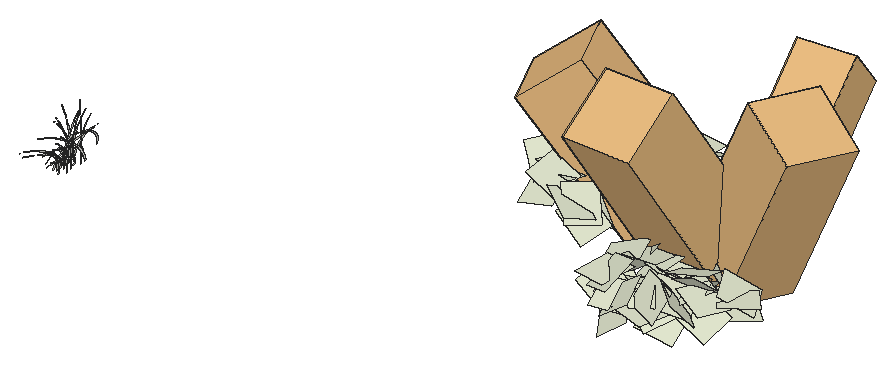
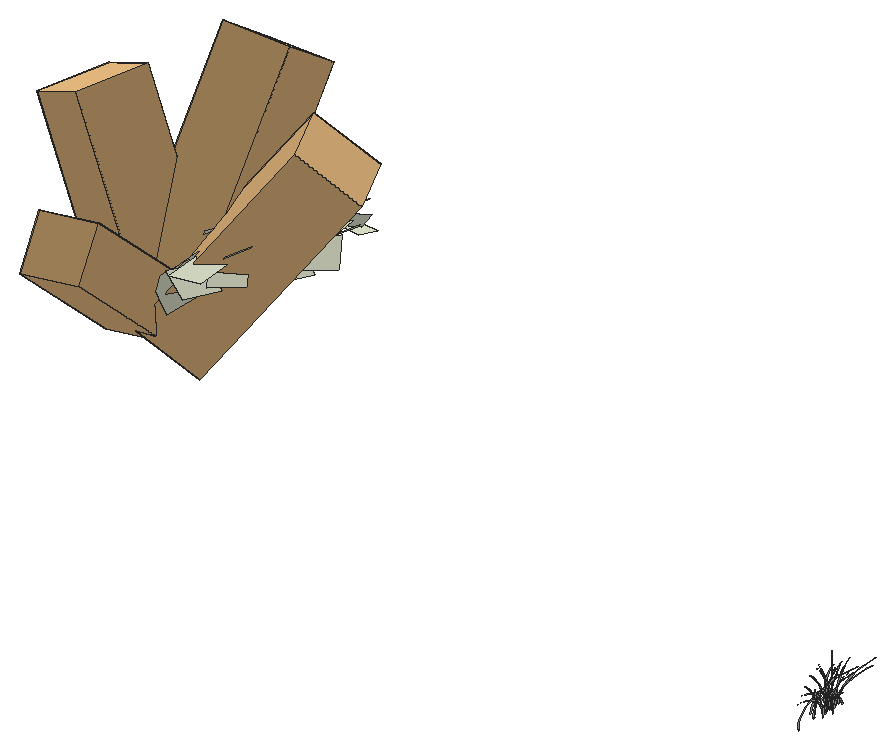
# SketchUp Ruby script. Lengths in inches.
U = 1.inch
M = Sketchup.active_model
def pt(a) = Geom::Point3d.new(a.map { |v| v * U })
def face(e, loops, mat)
  f = e.add_face(loops[0].map { |a| pt(a) })
  loops[1..].each { |l| e.add_face(l.map { |a| pt(a) }).erase! }
  f.material = f.back_material = mat if mat
  f
end
# faces: each face lists its corners as indices into pts; further lists are holes
def faces(e, pts, list, mat = nil) = list.each { |f| face(e, (f[0].is_a?(Array) ? f : [f]).map { |l| l.map { |i| pts[i] } }, mat) }
# xy, xz, yz: faces in a plane at the given z, y or x. An outline is a flat list of corners, or four numbers for a rectangle; further outlines are holes
def ring(l) = l.size == 4 ? [[l[0], l[1]], [l[2], l[1]], [l[2], l[3]], [l[0], l[3]]] : l.each_slice(2).to_a
def flat(e, list, mat, &to3) = list.each { |f| face(e, (f[0].is_a?(Array) ? f : [f]).map { |l| ring(l).map { |u, v| to3.(u, v) } }, mat) }
def xy(e, z, list, mat = nil) = flat(e, list, mat) { |x, y| [x, y, z] }
def xz(e, y, list, mat = nil) = flat(e, list, mat) { |x, z| [x, y, z] }
def yz(e, x, list, mat = nil) = flat(e, list, mat) { |y, z| [x, y, z] }
def lines(e, pts, list) = list.each { |a, b| e.add_line(pt(pts[a]), pt(pts[b])) }
# prism: a flat outline (further loops are holes) pulled along v
def prism(e, loops, v, mat = nil)
  f = face(e, loops, mat); d = Geom::Vector3d.new(v.map { |x| x * U })
  f.pushpull(f.normal.samedirection?(d) ? d.length : -d.length)
end
def box(e, o, s, mat = nil) = prism(e, [[o, [o[0] + s[0], o[1], o[2]], [o[0] + s[0], o[1] + s[1], o[2]], [o[0], o[1] + s[1], o[2]]]], [0, 0, s[2]], mat)
def at(x, y, z, deg = 0) = Geom::Transformation.translation(pt([x, y, z])) * Geom::Transformation.rotation(ORIGIN, Z_AXIS, deg.degrees)
def axes(o, x, y, z) = Geom::Transformation.new([*x, 0, *y, 0, *z, 0, *pt(o).to_a, 1])
def part(name) = M.definitions.add(name)
# library, detail: a bought-in or finely detailed component or shape, given as its bounding box
def library(name, o, s) = part(name).tap { |d| box(d.entities, o, s) }
def detail(e, o, s) = box(e.add_group.entities, o, s)
def put(e, d, t, mat = nil) = e.add_instance(d, t).tap { |i| i.material = mat if mat }
def group(e, t, mat = nil) = e.add_group.tap { |g| g.transformation = t; g.material = mat if mat }.entities
root = M.entities
M.materials.add("Celtis_australis_s cópia1").color = [224, 229, 205]
M.materials.add("bark_cherry").color = [99, 76, 62]
c1 = part("leaf1\#1")
p = [[1.6,6.78,0.04],[-9.34,-4.04,0.02],[2.67,-16.2,2.05],[13.62,-5.38,2.07]]
faces(c1.entities,p,[[0,1,2,3]],"Celtis_australis_s cópia1")
c2 = part("leaf_group1\#1")
put(c2.entities,c1,axes([-0.06,3.68,7.3125],[0.53029,-0.80282,-0.27253],[0.82812,0.42159,0.36943],[-0.18168,-0.42159,0.8884]))
put(c2.entities,c1,axes([6.4375,-3.58,5.23],[1,0,0],[0,0.98927,0.14608],[0,-0.14608,0.98927]))
put(c2.entities,c1,axes([-0.99,3.68,1.22],[0.57591,-0.80282,0.15431],[0.36532,0.42159,0.82994],[-0.73135,-0.42159,0.53609]))
put(c2.entities,c1,axes([18.71,8.59,4.39],[0.33053,0.77491,0.53877],[-0.79988,-0.073,0.5957],[0.50094,-0.62785,0.5957]))
put(c2.entities,c1,axes([13.16,0.76,0.89],[0.89618,0.3501,0.27256],[-0.44248,0.65988,0.60727],[0.03275,-0.66482,0.74628]))
put(c2.entities,c1,axes([4.53,7.98,7.3125],[-0.1927,0.94265,-0.27253],[0.88368,0.28746,0.36943],[-0.42658,0.16964,0.8884]))
put(c2.entities,c1,axes([12.46,21.28,7.16],[0.85019,0.38493,0.35918],[0.30538,-0.91629,0.25914],[-0.42887,0.11063,0.89657]))
put(c2.entities,c1,axes([6.53,15.18,2.59],[0.70711,0.70711,0],[0.5,-0.5,0.70711],[-0.5,0.5,0.70711]))
put(c2.entities,c1,axes([-3.17,8.15,3.46],[-0.03719,0.74973,0.66069],[0.94096,-0.19634,0.27576],[-0.33647,-0.63194,0.69817]))
put(c2.entities,c1,axes([23.03,17.79,4.39],[0.78166,-0.31422,0.53877],[-0.61722,-0.51398,0.5957],[-0.08973,0.79818,0.5957]))
put(c2.entities,c1,axes([14.78,21.52,3.21],[0.67246,-0.04394,0.73882],[-0.28657,-0.93583,0.20517],[-0.6824,0.3497,0.64191]))
put(c2.entities,c1,axes([10.37,-1.8125,9],[0.99279,-0.06448,-0.101],[0.11527,0.74421,0.65792],[0.03275,-0.66482,0.74628]))
put(c2.entities,c1,axes([1.45,16.1875,2.9375],[-0.2106,-0.86579,-0.45394],[0.96054,-0.26957,0.06852],[-0.18168,-0.42159,0.8884]))
c3 = library("branch1\#2",[0,0,0],[33.4,33.29,108.01])
c4 = part("branch2\#1")
p = [[13.74,0.36,0.5],[11.5,11.3125,10.98],[14.125,0.95,0],[14.97,0.95,0.19],[12.12,10.6875,11.67],[15.1,0.36,0.82],
  [11.05,10.4375,11.49],[14.34,0,1.01],[6.08,18.54,23.51],[6.83,18.32,23.89],[6.09,17.93,24.13],[3.27,29.37,34],
  [3.27,29.68,33.56],[3.73,29.59,33.82],[0,43.16,40.74],[0,43.16,40.75],[0.01,43.16,40.75],[5.59,23.2,32.77],
  [4.65,30.48,39.08],[1.92,39.79,43.02],[5.09,28.47,41.41]]
faces(c4.entities,p,[[0,1,2],[2,1,3],[3,4,5],[3,1,4],[6,0,7],[0,6,1],[5,6,7],[6,5,4],
  [6,8,1],[1,9,4],[9,1,8],[8,6,10],[4,10,6],[10,4,9],[10,11,8],[8,12,9],
  [12,8,11],[10,9,11],[13,11,9],[13,9,12],[14,12,11,15],[12,14,16,13],[13,16,15,11]],"bark_cherry")
lines(c4.entities,p,[[17,18],[11,19],[20,17],[17,10]])
g1 = group(root,at(29.53,759.15,-58.625))
p = [[-0.32,0.38,0],[-0.14,0.17,0],[0,0,1.28],[-0.06,0.07,2.5625],[-0.32,0.37,3.82],[-0.77,0.9,5.03],
  [-1.41,1.65,6.15],[-2.21,2.59,7.15],[-3.16,3.7,8.02],[-4.24,4.96,8.72],[-5.41,6.34,9.25],[-6.65,7.79,9.58],
  [-7.93,9.29,9.72],[-9.22,10.79,9.66],[-7.96,9.32,9.67],[-6.71,7.85,9.49],[-5.5,6.44,9.125],[-4.37,5.11,8.58],
  [-3.33,3.89,7.87],[-2.4,2.8125,7.01],[-1.62,1.9,6.02],[-1,1.17,4.92],[-0.55,0.65,3.75],[-0.29,0.33,2.51],
  [-0.21,0.24,1.26]]
faces(g1,p,[[0,1,2,3,4,5,6,7,8,9,10,11,12,13,14,15,16,17,18,19,20,21,22,23,24]])
g2 = group(root,at(25.89,760.17,-58.625))
p = [[-1.7,3.48,4.89],[-1.39,2.85,4.58],[-1.11,2.27,4.24],[-0.86,1.76,3.875],[-0.65,1.33,3.48],[-0.47,0.96,3.08],
  [-0.33,0.68,2.65],[-0.23,0.48,2.22],[-0.18,0.36,1.77],[-0.16,0.33,1.32],[-0.18,0.38,0.875],[-0.25,0.51,0.43],
  [-0.36,0.73,0],[-0.22,0.45,0],[-0.1,0.21,0.44],[-0.03,0.06,0.89],[0,0,1.35],[-0.02,0.04,1.8],
  [-0.08,0.17,2.25],[-0.19,0.4,2.7],[-0.35,0.71,3.125],[-0.54,1.11,3.53],[-0.78,1.6,3.92],[-1.05,2.16,4.27],
  [-1.36,2.79,4.6]]
faces(g2,p,[[0,1,2,3,4,5,6,7,8,9,10,11,12,13,14,15,16,17,18,19,20,21,22,23,24]])
g3 = group(root,at(29.06,755.59,-58.625))
p = [[-0.27,0.46,0],[-0.12,0.21,0],[0,0,1.09],[-0.05,0.08,2.18],[-0.26,0.45,3.25],[-0.64,1.1,4.27],
  [-1.16,2.02,5.22],[-1.82,3.17,6.08],[-2.61,4.53,6.8125],[-3.49,6.07,7.41],[-4.46,7.76,7.86],[-5.48,9.53,8.15],
  [-6.54,11.37,8.26],[-7.59,13.21,8.21],[-6.56,11.4,8.22],[-5.53,9.61,8.07],[-4.53,7.89,7.76],[-3.6,6.26,7.29],
  [-2.74,4.77,6.69],[-1.98,3.44,5.96],[-1.34,2.33,5.12],[-0.82,1.43,4.1875],[-0.45,0.79,3.18],[-0.24,0.41,2.14],
  [-0.17,0.3,1.07]]
faces(g3,p,[[0,1,2,3,4,5,6,7,8,9,10,11,12,13,14,15,16,17,18,19,20,21,22,23,24]])
g4 = group(root,at(27.63,757.12,-58.625))
p = [[-0.51,0.05,0],[-0.23,0.02,0.96],[-0.06,0.01,1.92],[0,0,2.9],[-0.06,0.01,3.87],[-0.22,0.02,4.83],
  [-0.51,0.05,5.79],[-0.9,0.09,6.74],[-1.4,0.14,7.67],[-2,0.2,8.57],[-2.72,0.27,9.46],[-3.53,0.35,10.3125],
  [-4.44,0.44,11.13],[-3.58,0.35,10.3],[-2.82,0.28,9.43],[-2.14,0.21,8.55],[-1.5625,0.15,7.64],[-1.08,0.11,6.71],
  [-0.69,0.07,5.77],[-0.41,0.04,4.82],[-0.23,0.02,3.86],[-0.14,0.01,2.89],[-0.16,0.02,1.92],[-0.29,0.03,0.96]]
faces(g4,p,[[0,1,2,3,4,5,6,7,8,9,10,11,12,13,14,15,16,17,18,19,20,21,22,23]])
g5 = group(root,at(26.74,754.9375,-58.625))
p = [[-2.09,-11.02,8.28],[-2.4,-12.68,8.5],[-2.1,-11.07,8.24],[-1.8,-9.52,7.87],[-1.52,-8.03,7.41],[-1.26,-6.64,6.85],
  [-1.01,-5.35,6.21],[-0.79,-4.18,5.49],[-0.6,-3.14,4.69],[-0.43,-2.25,3.84],[-0.29,-1.51,2.93],[-0.18,-0.93,1.98],
  [-0.1,-0.52,1],[-0.05,-0.29,0],[0,0,0],[-0.04,-0.19,1.03],[-0.11,-0.58,2.03],[-0.22,-1.15,3],
  [-0.36,-1.89,3.93],[-0.53,-2.8,4.8],[-0.73,-3.87,5.61],[-0.96,-5.08,6.33],[-1.22,-6.42,6.97],[-1.49,-7.87,7.51],
  [-1.78,-9.41,7.95]]
faces(g5,p,[[0,1,2,3,4,5,6,7,8,9,10,11,12,13,14,15,16,17,18,19,20,21,22,23,24]])
g6 = group(root,at(26.9375,755.96,-58.625))
p = [[-2.09,-11.02,6.68],[-2.4,-12.68,6.86],[-2.1,-11.07,6.64],[-1.8,-9.52,6.35],[-1.52,-8.03,5.97],[-1.26,-6.64,5.52],
  [-1.01,-5.35,5.01],[-0.79,-4.18,4.42],[-0.6,-3.14,3.79],[-0.43,-2.25,3.1],[-0.29,-1.51,2.36],[-0.18,-0.93,1.6],
  [-0.1,-0.52,0.81],[-0.05,-0.29,0],[0,0,0],[-0.04,-0.19,0.83],[-0.11,-0.58,1.64],[-0.22,-1.15,2.42],
  [-0.36,-1.89,3.17],[-0.53,-2.8,3.875],[-0.73,-3.87,4.52],[-0.96,-5.08,5.11],[-1.22,-6.42,5.62],[-1.49,-7.87,6.06],
  [-1.78,-9.41,6.41]]
faces(g6,p,[[0,1,2,3,4,5,6,7,8,9,10,11,12,13,14,15,16,17,18,19,20,21,22,23,24]])
g7 = group(root,at(26.97,759.05,-58.625))
p = [[-2.3,-4.58,4.26],[-1.86,-3.71,3.98],[-1.47,-2.92,3.6875],[-1.12,-2.22,3.37],[-0.82,-1.625,3.03],[-0.57,-1.13,2.68],
  [-0.375,-0.75,2.31],[-0.24,-0.47,1.93],[-0.15,-0.31,1.54],[-0.13,-0.26,1.15],[-0.17,-0.33,0.76],[-0.26,-0.51,0.38],
  [-0.41,-0.8125,0],[-0.31,-0.61,0],[-0.14,-0.27,0.375],[-0.03,-0.06,0.76],[0.01,0.03,1.15],[0,-0.01,1.54],
  [-0.09,-0.18,1.93],[-0.23,-0.47,2.32],[-0.44,-0.88,2.6875],[-0.71,-1.41,3.05],[-1.03,-2.05,3.39],[-1.41,-2.8,3.7],
  [-1.83,-3.65,3.99]]
faces(g7,p,[[0,1,2,3,4,5,6,7,8,9,10,11,12,13,14,15,16,17,18,19,20,21,22,23,24]])
g8 = group(root,at(28.05,757.3125,-58.625))
p = [[-0.48,0.17,0],[-0.21,0.08,1.22],[-0.05,0.02,2.46],[0,0,3.69],[-0.05,0.02,4.93],[-0.21,0.08,6.17],
  [-0.48,0.17,7.39],[-0.85,0.31,8.6],[-1.32,0.48,9.78],[-1.89,0.6875,10.9375],[-2.57,0.93,12.07],[-3.33,1.21,13.16],
  [-4.19,1.52,14.2],[-3.39,1.23,13.14],[-2.66,0.96,12.04],[-2.02,0.73,10.91],[-1.47,0.53,9.75],[-1.02,0.37,8.5625],
  [-0.66,0.24,7.36],[-0.39,0.14,6.15],[-0.21,0.08,4.92],[-0.14,0.05,3.6875],[-0.15,0.06,2.45],[-0.27,0.1,1.22]]
faces(g8,p,[[0,1,2,3,4,5,6,7,8,9,10,11,12,13,14,15,16,17,18,19,20,21,22,23]])
g9 = group(root,at(27.07,758.11,-58.625))
p = [[-0.22,-0.46,0],[-0.1,-0.21,1.0625],[-0.02,-0.05,2.14],[0,0,3.21],[-0.02,-0.05,4.29],[-0.1,-0.2,5.36],
  [-0.22,-0.46,6.43],[-0.39,-0.8125,7.48],[-0.6,-1.27,8.51],[-0.87,-1.82,9.52],[-1.18,-2.46,10.5],[-1.53,-3.2,11.45],
  [-1.92,-4.03,12.36],[-1.55,-3.25,11.43],[-1.22,-2.55,10.47],[-0.93,-1.94,9.49],[-0.68,-1.42,8.48],[-0.47,-0.98,7.45],
  [-0.3,-0.63,6.4],[-0.18,-0.37,5.35],[-0.1,-0.2,4.28],[-0.0625,-0.13,3.21],[-0.07,-0.15,2.13],[-0.125,-0.26,1.0625]]
faces(g9,p,[[0,1,2,3,4,5,6,7,8,9,10,11,12,13,14,15,16,17,18,19,20,21,22,23]])
g10 = group(root,at(26.16,759.5,-58.625))
p = [[0.03,-0.41,0],[0.01,-0.18,0],[0,0,0.79],[0,-0.07,1.58],[0.03,-0.4,2.36],[0.0625,-0.97,3.11],
  [0.11,-1.77,3.8],[0.18,-2.79,4.42],[0.26,-3.99,4.95],[0.35,-5.34,5.39],[0.44,-6.82,5.71],[0.54,-8.38,5.92],
  [0.65,-9.99,6.01],[0.75,-11.61,5.96],[0.65,-10.02,5.97],[0.55,-8.45,5.86],[0.45,-6.93,5.64],[0.36,-5.5,5.3],
  [0.27,-4.19,4.86],[0.2,-3.03,4.33],[0.13,-2.04,3.72],[0.08,-1.26,3.04],[0.04,-0.69,2.3125],[0.02,-0.36,1.55],
  [0.02,-0.26,0.78]]
faces(g10,p,[[0,1,2,3,4,5,6,7,8,9,10,11,12,13,14,15,16,17,18,19,20,21,22,23,24]])
g11 = group(root,at(26.16,759.5,-58.625))
p = [[0.03,-0.41,0],[0.01,-0.18,0],[0,0,0.79],[0,-0.07,1.58],[0.03,-0.4,2.36],[0.0625,-0.97,3.11],
  [0.11,-1.77,3.8],[0.18,-2.79,4.42],[0.26,-3.99,4.95],[0.35,-5.34,5.39],[0.44,-6.82,5.71],[0.54,-8.38,5.92],
  [0.65,-9.99,6.01],[0.75,-11.61,5.96],[0.65,-10.02,5.97],[0.55,-8.45,5.86],[0.45,-6.93,5.64],[0.36,-5.5,5.3],
  [0.27,-4.19,4.86],[0.2,-3.03,4.33],[0.13,-2.04,3.72],[0.08,-1.26,3.04],[0.04,-0.69,2.3125],[0.02,-0.36,1.55],
  [0.02,-0.26,0.78]]
faces(g11,p,[[0,1,2,3,4,5,6,7,8,9,10,11,12,13,14,15,16,17,18,19,20,21,22,23,24]])
g12 = group(root,at(26.17,769.54,-58.625))
p = [[0.03,-0.46,0],[0.01,-0.21,0],[0,0,0.89],[0.01,-0.08,1.79],[0.03,-0.45,2.67],[0.07,-1.1,3.51],
  [0.13,-2,4.29],[0.2,-3.15,4.99],[0.29,-4.5,5.59],[0.39,-6.04,6.09],[0.5,-7.71,6.45],[0.61,-9.47,6.69],
  [0.73,-11.29,6.79],[0.85,-13.12,6.74],[0.73,-11.33,6.75],[0.62,-9.55,6.625],[0.51,-7.84,6.37],[0.4,-6.22,5.99],
  [0.31,-4.73,5.49],[0.22,-3.42,4.89],[0.15,-2.31,4.2],[0.09,-1.42,3.4375],[0.05,-0.78,2.62],[0.03,-0.41,1.75],
  [0.02,-0.3,0.875]]
faces(g12,p,[[0,1,2,3,4,5,6,7,8,9,10,11,12,13,14,15,16,17,18,19,20,21,22,23,24]])
g13 = group(root,at(28.97,757.5,-58.625))
p = [[-4.78,1.84,4.89],[-3.87,1.49,4.58],[-3.05,1.18,4.24],[-2.32,0.9,3.875],[-1.7,0.66,3.48],[-1.18,0.46,3.08],
  [-0.78,0.3,2.65],[-0.49,0.1875,2.22],[-0.32,0.125,1.77],[-0.27,0.11,1.32],[-0.34,0.13,0.875],[-0.54,0.21,0.43],
  [-0.85,0.33,0],[-0.64,0.25,0],[-0.29,0.11,0.43],[-0.0625,0.02,0.87],[0.03,-0.01,1.32],[-0.01,0,1.77],
  [-0.18,0.07,2.22],[-0.49,0.1875,2.66],[-0.92,0.35,3.09],[-1.47,0.57,3.5],[-2.15,0.83,3.89],[-2.93,1.13,4.26],
  [-3.81,1.47,4.59]]
faces(g13,p,[[0,1,2,3,4,5,6,7,8,9,10,11,12,13,14,15,16,17,18,19,20,21,22,23,24]])
g14 = group(root,at(29.09,761.39,-58.625))
p = [[-4.27,-10.37,9.03],[-4.92,-11.93,9.27],[-4.29,-10.42,8.98],[-3.69,-8.96,8.58],[-3.12,-7.56,8.08],[-2.58,-6.25,7.47],
  [-2.08,-5.04,6.77],[-1.62,-3.94,5.98],[-1.22,-2.96,5.12],[-0.87,-2.12,4.1875],[-0.59,-1.42,3.2],[-0.36,-0.88,2.16],
  [-0.2,-0.49,1.09],[-0.11,-0.27,0],[0,0,0],[-0.08,-0.18,1.12],[-0.22,-0.54,2.22],[-0.44,-1.08,3.28],
  [-0.73,-1.78,4.29],[-1.09,-2.64,5.24],[-1.5,-3.64,6.11],[-1.97,-4.78,6.9],[-2.49,-6.04,7.6],[-3.05,-7.4,8.19],
  [-3.65,-8.85,8.67]]
faces(g14,p,[[0,1,2,3,4,5,6,7,8,9,10,11,12,13,14,15,16,17,18,19,20,21,22,23,24]])
g15 = group(root,at(27.12,759.32,-58.625))
yz(g15,0,[[0.08,0,0,0.81,0.11,1.62,0.4,2.41,0.87,3.16,1.5,3.85,2.29,4.48,3.22,5.03,4.26,5.47,5.39,5.82,6.58,6.04,7.82,6.15,9.07,6.14,7.85,6.1,6.65,5.95,5.49,5.7,4.4,5.34,3.4,4.89,2.5,4.36,1.72,3.74,1.08,3.07,0.58,2.34,0.25,1.58,0.08,0.79]])
g16 = group(root,at(27.12,756.66,-58.625))
yz(g16,0,[[0.51,0,0.23,1.1,0.06,2.21,0,3.33,0.06,4.44,0.23,5.56,0.51,6.66,0.9,7.74,1.4,8.8125,2.01,9.85,2.73,10.87,3.55,11.85,4.46,12.8,3.6,11.84,2.83,10.84,2.15,9.82,1.57,8.78,1.08,7.71,0.7,6.63,0.41,5.54,0.23,4.43,0.14,3.32,0.16,2.21,0.29,1.1]])
g17 = group(root,at(27.12,758.1,-58.625))
yz(g17,0,[[0.07,0,0,1.08,0.03,2.17,0.16,3.25,0.39,4.32,0.72,5.38,1.16,6.43,1.6875,7.46,2.31,8.46,3.04,9.4375,3.85,10.38,4.75,11.29,5.73,12.17,4.82,11.27,3.98,10.34,3.22,9.39,2.53,8.4,1.93,7.4,1.41,6.38,0.97,5.34,0.62,4.29,0.35,3.22,0.17,2.15,0.08,1.08]])
g18 = group(root,at(27.12,761.76,-58.625))
yz(g18,0,[[0.5,0,0.23,0.89,0.0625,1.81,0,2.74,0.04,3.66,0.19,4.58,0.44,5.48,0.79,6.35,1.24,7.18,1.78,7.96,2.4,8.69,3.1,9.35,3.875,9.94,3.17,9.3125,2.53,8.62,1.96,7.875,1.48,7.08,1.07,6.25,0.76,5.39,0.53,4.5,0.4,3.6,0.36,2.69,0.42,1.78,0.57,0.88,0.8125,0]])
g19 = group(root,at(26.76,753.74,-58.625))
p = [[0.78,-3.8,3.62],[0.64,-3.1,3.39],[0.51,-2.47,3.14],[0.4,-1.92,2.86],[0.3,-1.44,2.58],[0.22,-1.05,2.27],
  [0.15,-0.74,1.96],[0.11,-0.52,1.64],[0.08,-0.39,1.31],[0.07,-0.36,0.98],[0.08,-0.41,0.65],[0.12,-0.56,0.32],
  [0.16,-0.79,0],[0.1,-0.49,0],[0.05,-0.22,0.33],[0.01,-0.0625,0.66],[0,0,1],[0.01,-0.04,1.33],
  [0.04,-0.1875,1.67],[0.09,-0.43,1.99],[0.16,-0.77,2.31],[0.25,-1.21,2.61],[0.36,-1.74,2.9],[0.49,-2.35,3.16],
  [0.63,-3.04,3.4]]
faces(g19,p,[[0,1,2,3,4,5,6,7,8,9,10,11,12,13,14,15,16,17,18,19,20,21,22,23,24]])
g20 = group(root,at(26.04,752.64,-58.625))
p = [[2.09,11.02,6.68],[2.4,12.68,6.86],[2.1,11.07,6.64],[1.8,9.52,6.35],[1.52,8.03,5.97],[1.26,6.64,5.52],
  [1.01,5.35,5.01],[0.79,4.18,4.42],[0.6,3.14,3.79],[0.43,2.25,3.1],[0.29,1.51,2.36],[0.18,0.93,1.6],
  [0.1,0.52,0.81],[0.05,0.29,0],[0,0,0],[0.04,0.19,0.83],[0.11,0.58,1.64],[0.22,1.15,2.42],
  [0.36,1.89,3.17],[0.53,2.8,3.875],[0.73,3.87,4.52],[0.96,5.08,5.11],[1.22,6.42,5.62],[1.49,7.87,6.06],
  [1.78,9.41,6.41]]
faces(g20,p,[[0,1,2,3,4,5,6,7,8,9,10,11,12,13,14,15,16,17,18,19,20,21,22,23,24]])
g21 = group(root,at(26.86,763.03,-58.625))
p = [[0.89,-4.29,4.09],[0.72,-3.5,3.83],[0.58,-2.8,3.54],[0.45,-2.17,3.24],[0.34,-1.63,2.91],[0.25,-1.1875,2.57],
  [0.17,-0.84,2.22],[0.12,-0.59,1.85],[0.09,-0.44,1.48],[0.08,-0.4,1.11],[0.1,-0.46,0.73],[0.13,-0.63,0.36],
  [0.19,-0.9,0],[0.11,-0.55,0],[0.05,-0.25,0.37],[0.01,-0.07,0.74],[0,0,1.125],[0.01,-0.05,1.51],
  [0.04,-0.21,1.88],[0.1,-0.49,2.25],[0.18,-0.875,2.61],[0.28,-1.37,2.95],[0.41,-1.96,3.27],[0.55,-2.65,3.57],
  [0.71,-3.43,3.84]]
faces(g21,p,[[0,1,2,3,4,5,6,7,8,9,10,11,12,13,14,15,16,17,18,19,20,21,22,23,24]])
g22 = group(root,at(27.02,757.67,-58.625))
p = [[0.1,-0.5,0],[0.05,-0.22,0.8125],[0.01,-0.06,1.64],[0,0,2.46],[0.01,-0.05,3.29],[0.05,-0.22,4.11],
  [0.1,-0.5,4.92],[0.18,-0.88,5.73],[0.28,-1.375,6.52],[0.41,-1.97,7.29],[0.55,-2.67,8.04],[0.72,-3.47,8.76],
  [0.9,-4.37,9.46],[0.73,-3.53,8.75],[0.57,-2.77,8.02],[0.44,-2.11,7.27],[0.32,-1.54,6.49],[0.22,-1.0625,5.7],
  [0.14,-0.68,4.9],[0.08,-0.4,4.09],[0.05,-0.22,3.28],[0.03,-0.14,2.46],[0.03,-0.16,1.63],[0.06,-0.28,0.81]]
faces(g22,p,[[0,1,2,3,4,5,6,7,8,9,10,11,12,13,14,15,16,17,18,19,20,21,22,23]])
g23 = group(root,at(24.88,758.11,-58.625))
p = [[0.21,-0.49,0],[0.09,-0.22,0],[0,0,0.95],[0.04,-0.09,1.9],[0.21,-0.48,2.83],[0.5,-1.17,3.72],
  [0.91,-2.14,4.55],[1.43,-3.36,5.29],[2.05,-4.81,5.93],[2.75,-6.45,6.45],[3.51,-8.23,6.84],[4.31,-10.12,7.09],
  [5.14,-12.06,7.1875],[5.98,-14.01,7.14],[5.16,-12.1,7.15],[4.35,-10.2,7.02],[3.57,-8.37,6.75],[2.83,-6.64,6.35],
  [2.16,-5.06,5.82],[1.56,-3.65,5.18],[1.05,-2.47,4.45],[0.65,-1.52,3.64],[0.36,-0.84,2.77],[0.19,-0.43,1.86],
  [0.14,-0.32,0.93]]
faces(g23,p,[[0,1,2,3,4,5,6,7,8,9,10,11,12,13,14,15,16,17,18,19,20,21,22,23,24]])
g24 = group(root,at(25.37,756.47,-58.625))
p = [[5.05,-0.84,3.62],[4.09,-0.68,3.39],[3.22,-0.54,3.14],[2.46,-0.41,2.86],[1.8,-0.3,2.58],[1.25,-0.21,2.27],
  [0.82,-0.14,1.96],[0.52,-0.09,1.64],[0.34,-0.06,1.31],[0.29,-0.05,0.98],[0.36,-0.06,0.65],[0.57,-0.09,0.32],
  [0.9,-0.15,0],[0.68,-0.11,0],[0.3,-0.05,0.32],[0.07,-0.01,0.64],[-0.03,0.01,0.98],[0.01,0,1.31],
  [0.19,-0.03,1.64],[0.52,-0.09,1.97],[0.97,-0.16,2.28],[1.56,-0.26,2.59],[2.27,-0.375,2.88],[3.09,-0.51,3.15],
  [4.03,-0.67,3.39]]
faces(g24,p,[[0,1,2,3,4,5,6,7,8,9,10,11,12,13,14,15,16,17,18,19,20,21,22,23,24]])
g25 = group(root,at(27.31,756.27,-58.625))
p = [[1.16,-5.61,9],[0.98,-4.72,8.33],[0.81,-3.9,7.65],[0.65,-3.15,6.94],[0.51,-2.48,6.22],[0.39,-1.89,5.47],
  [0.28,-1.375,4.72],[0.2,-0.95,3.95],[0.125,-0.6,3.17],[0.07,-0.34,2.38],[0.03,-0.17,1.59],[0.02,-0.08,0.8],
  [0.02,-0.07,0],[0,0,0.8],[0.01,-0.03,1.6],[0.03,-0.15,2.4],[0.08,-0.38,3.19],[0.15,-0.71,3.98],
  [0.23,-1.13,4.75],[0.34,-1.65,5.51],[0.47,-2.27,6.26],[0.61,-2.97,6.98],[0.78,-3.77,7.68],[0.96,-4.65,8.35]]
faces(g25,p,[[0,1,2,3,4,5,6,7,8,9,10,11,12,13,14,15,16,17,18,19,20,21,22,23]])
g26 = group(root,at(28.05,752.68,-58.625))
p = [[0.78,-3.8,7.35],[0.64,-3.1,6.89],[0.51,-2.47,6.375],[0.4,-1.92,5.82],[0.3,-1.44,5.24],[0.22,-1.05,4.625],
  [0.15,-0.74,3.99],[0.11,-0.52,3.33],[0.08,-0.39,2.66],[0.07,-0.36,1.99],[0.08,-0.41,1.32],[0.12,-0.56,0.65],
  [0.16,-0.79,0],[0.1,-0.49,0],[0.05,-0.22,0.66],[0.01,-0.0625,1.34],[0,0,2.02],[0.01,-0.04,2.71],
  [0.04,-0.1875,3.39],[0.09,-0.43,4.05],[0.16,-0.77,4.7],[0.25,-1.21,5.31],[0.36,-1.74,5.89],[0.49,-2.35,6.43],
  [0.63,-3.04,6.92]]
faces(g26,p,[[0,1,2,3,4,5,6,7,8,9,10,11,12,13,14,15,16,17,18,19,20,21,22,23,24]])
g27 = group(root,at(26.24,756.84,-58.625))
p = [[0.51,-0.07,0],[0.23,-0.03,0.9],[0.06,-0.01,1.82],[0,0,2.73],[0.06,-0.01,3.65],[0.22,-0.03,4.56],
  [0.5,-0.07,5.46],[0.89,-0.13,6.36],[1.39,-0.2,7.23],[1.99,-0.29,8.09],[2.7,-0.39,8.92],[3.51,-0.51,9.73],
  [4.42,-0.64,10.5],[3.5625,-0.51,9.72],[2.8,-0.4,8.9],[2.13,-0.31,8.0625],[1.55,-0.22,7.21],[1.07,-0.15,6.33],
  [0.69,-0.1,5.44],[0.41,-0.06,4.54],[0.22,-0.03,3.64],[0.14,-0.02,2.73],[0.16,-0.02,1.8125],[0.28,-0.04,0.9]]
faces(g27,p,[[0,1,2,3,4,5,6,7,8,9,10,11,12,13,14,15,16,17,18,19,20,21,22,23]])
g28 = group(root,at(27.55,755.0625,-58.625))
p = [[1.84,-8.88,4.54],[1.59,-7.6875,4.51],[1.35,-6.51,4.4],[1.11,-5.38,4.21],[0.89,-4.31,3.95],[0.6875,-3.33,3.62],
  [0.51,-2.44,3.22],[0.35,-1.68,2.77],[0.22,-1.05,2.27],[0.12,-0.57,1.73],[0.05,-0.24,1.17],[0.02,-0.08,0.59],
  [0.02,-0.08,0],[0,0,0.6],[0.02,-0.1,1.2],[0.08,-0.39,1.78],[0.18,-0.85,2.33],[0.3,-1.47,2.85],
  [0.46,-2.24,3.3125],[0.65,-3.15,3.72],[0.86,-4.17,4.05],[1.09,-5.28,4.3],[1.33,-6.45,4.47],[1.58,-7.66,4.55]]
faces(g28,p,[[0,1,2,3,4,5,6,7,8,9,10,11,12,13,14,15,16,17,18,19,20,21,22,23]])
g29 = group(root,at(28.93,754.48,-58.625))
p = [[2.37,-3.07,3.62],[1.9375,-2.51,3.39],[1.54,-2,3.14],[1.2,-1.55,2.86],[0.9,-1.17,2.58],[0.66,-0.85,2.27],
  [0.46,-0.6,1.96],[0.33,-0.42,1.64],[0.25,-0.32,1.31],[0.22,-0.29,0.98],[0.26,-0.33,0.65],[0.35,-0.45,0.32],
  [0.5,-0.64,0],[0.3,-0.39,0],[0.14,-0.18,0.33],[0.04,-0.05,0.66],[0,0,1],[0.03,-0.03,1.33],
  [0.12,-0.15,1.67],[0.27,-0.35,1.99],[0.48,-0.625,2.31],[0.76,-0.98,2.61],[1.09,-1.41,2.9],[1.47,-1.9,3.16],
  [1.9,-2.45,3.4]]
faces(g29,p,[[0,1,2,3,4,5,6,7,8,9,10,11,12,13,14,15,16,17,18,19,20,21,22,23,24]])
g30 = group(root,at(25.99,756.8125,-58.625))
p = [[0.3125,-0.39,0],[0.14,-0.17,0],[0,0,1.11],[0.06,-0.07,2.23],[0.31,-0.38,3.33],[0.74,-0.93,4.375],
  [1.36,-1.69,5.35],[2.13,-2.66,6.22],[3.05,-3.8,6.97],[4.08,-5.09,7.59],[5.21,-6.5,8.05],[6.41,-8,8.34],
  [7.64,-9.53,8.46],[8.87,-11.07,8.4],[7.66,-9.5625,8.41],[6.46,-8.0625,8.26],[5.3,-6.61,7.9375],[4.2,-5.25,7.47],
  [3.2,-4,6.85],[2.3125,-2.89,6.1],[1.5625,-1.95,5.24],[0.96,-1.2,4.28],[0.53,-0.66,3.26],[0.27,-0.34,2.1875],
  [0.2,-0.25,1.09]]
faces(g30,p,[[0,1,2,3,4,5,6,7,8,9,10,11,12,13,14,15,16,17,18,19,20,21,22,23,24]])
g31 = group(root,at(25.99,756.8125,-58.625))
p = [[0.3125,-0.39,0],[0.14,-0.17,0],[0,0,1.11],[0.06,-0.07,2.23],[0.31,-0.38,3.33],[0.74,-0.93,4.375],
  [1.36,-1.69,5.35],[2.13,-2.66,6.22],[3.05,-3.8,6.97],[4.08,-5.09,7.59],[5.21,-6.5,8.05],[6.41,-8,8.34],
  [7.64,-9.53,8.46],[8.87,-11.07,8.4],[7.66,-9.5625,8.41],[6.46,-8.0625,8.26],[5.3,-6.61,7.9375],[4.2,-5.25,7.47],
  [3.2,-4,6.85],[2.3125,-2.89,6.1],[1.5625,-1.95,5.24],[0.96,-1.2,4.28],[0.53,-0.66,3.26],[0.27,-0.34,2.1875],
  [0.2,-0.25,1.09]]
faces(g31,p,[[0,1,2,3,4,5,6,7,8,9,10,11,12,13,14,15,16,17,18,19,20,21,22,23,24]])
put(root,c2,axes([193.78,732.5625,4.33],[0.45516,0.2017,-0.35249],[-0.24714,0.55769,0],[0.32227,0.14281,0.49784]))
put(root,c3,axes([209.51,767.69,-28.26],[0.26995,-0.54686,0.0132],[0.43326,0.22274,0.36711],[-0.33393,-0.15308,0.48699]))
put(root,c2,axes([205.98,752.58,4.33],[0.45516,0.2017,-0.35249],[-0.24714,0.55769,0],[0.32227,0.14281,0.49784]))
put(root,c3,axes([212.71,750.34,-20.98],[0.61,0,0],[0,0.50272,0.34551],[0,-0.34551,0.50272]))
put(root,c2,axes([221.31,724.17,-15.24],[0.51021,0.32254,-0.08806],[-0.32595,0.51561,0],[0.07443,0.04705,0.60361]))
put(root,c3,axes([235.31,771.18,-21.77],[-0.47472,-0.08003,0.02144],[0.06828,-0.30726,0.36491],[-0.04693,0.36251,0.31402]))
put(root,c4,axes([217.97,760.01,-20.42],[0.5929,0.14344,0],[0.12946,-0.53514,-0.26261],[0.06175,-0.25525,0.55058]))
put(root,c2,axes([217.43,731.78,-8.64],[0.36326,-0.48206,-0.08806],[0.48717,0.36711,0],[0.05299,-0.07033,0.60361]))
put(root,c2,axes([240.95,732.33,-12.52],[0.02633,0.60304,-0.08806],[-0.60942,0.02661,0],[0.00384,0.08797,0.60361]))
put(root,c3,axes([235.64,744.63,-19.47],[0.19859,0.57478,-0.04786],[-0.51441,0.1994,0.26024],[0.2139,-0.03638,0.45069]))
